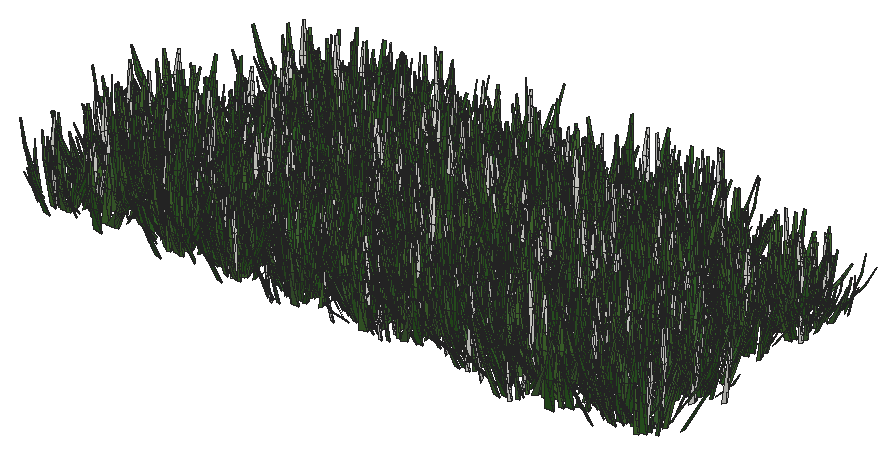
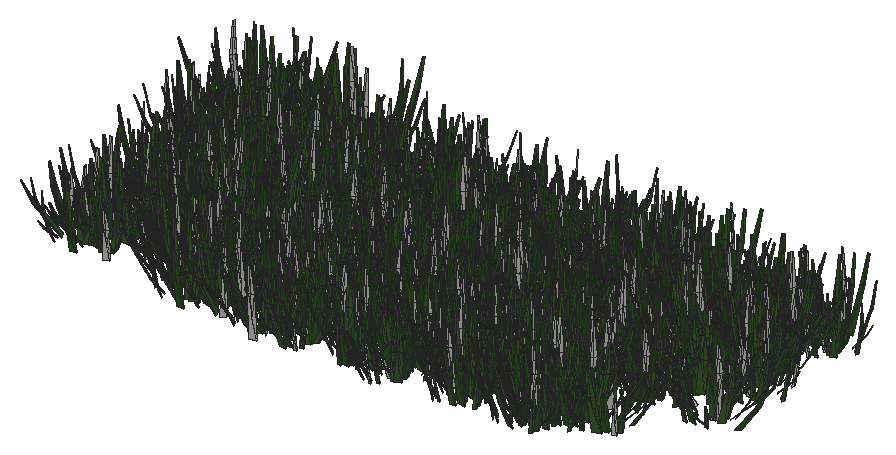
# SketchUp Ruby script. Lengths in inches.
U = 1.inch
M = Sketchup.active_model
def pt(a) = Geom::Point3d.new(a.map { |v| v * U })
def face(e, loops, mat)
  f = e.add_face(loops[0].map { |a| pt(a) })
  loops[1..].each { |l| e.add_face(l.map { |a| pt(a) }).erase! }
  f.material = f.back_material = mat if mat
  f
end
# faces: each face lists its corners as indices into pts; further lists are holes
def faces(e, pts, list, mat = nil) = list.each { |f| face(e, (f[0].is_a?(Array) ? f : [f]).map { |l| l.map { |i| pts[i] } }, mat) }
# xy, xz, yz: faces in a plane at the given z, y or x. An outline is a flat list of corners, or four numbers for a rectangle; further outlines are holes
def ring(l) = l.size == 4 ? [[l[0], l[1]], [l[2], l[1]], [l[2], l[3]], [l[0], l[3]]] : l.each_slice(2).to_a
def flat(e, list, mat, &to3) = list.each { |f| face(e, (f[0].is_a?(Array) ? f : [f]).map { |l| ring(l).map { |u, v| to3.(u, v) } }, mat) }
def xy(e, z, list, mat = nil) = flat(e, list, mat) { |x, y| [x, y, z] }
def xz(e, y, list, mat = nil) = flat(e, list, mat) { |x, z| [x, y, z] }
def yz(e, x, list, mat = nil) = flat(e, list, mat) { |y, z| [x, y, z] }
def lines(e, pts, list) = list.each { |a, b| e.add_line(pt(pts[a]), pt(pts[b])) }
# prism: a flat outline (further loops are holes) pulled along v
def prism(e, loops, v, mat = nil)
  f = face(e, loops, mat); d = Geom::Vector3d.new(v.map { |x| x * U })
  f.pushpull(f.normal.samedirection?(d) ? d.length : -d.length)
end
def box(e, o, s, mat = nil) = prism(e, [[o, [o[0] + s[0], o[1], o[2]], [o[0] + s[0], o[1] + s[1], o[2]], [o[0], o[1] + s[1], o[2]]]], [0, 0, s[2]], mat)
def at(x, y, z, deg = 0) = Geom::Transformation.translation(pt([x, y, z])) * Geom::Transformation.rotation(ORIGIN, Z_AXIS, deg.degrees)
def axes(o, x, y, z) = Geom::Transformation.new([*x, 0, *y, 0, *z, 0, *pt(o).to_a, 1])
def part(name) = M.definitions.add(name)
# library, detail: a bought-in or finely detailed component or shape, given as its bounding box
def library(name, o, s) = part(name).tap { |d| box(d.entities, o, s) }
def detail(e, o, s) = box(e.add_group.entities, o, s)
def put(e, d, t, mat = nil) = e.add_instance(d, t).tap { |i| i.material = mat if mat }
def group(e, t, mat = nil) = e.add_group.tap { |g| g.transformation = t; g.material = mat if mat }.entities
root = M.entities
M.materials.add("Material1").color = [58, 110, 58]
M.materials.add("Material10").color = [48, 100, 38]
M.materials.add("Material3").color = [68, 110, 58]
M.materials.add("Material4").color = [48, 90, 38]
M.materials.add("Material5").color = [68, 110, 48]
M.materials.add("Material6").color = [48, 90, 48]
M.materials.add("Material8").color = [58, 90, 38]
M.materials.add("Material9").color = [68, 100, 58]
c1 = part("grass00")
p = [[-0.6875,0.15,0],[-0.56,0.08,5.52],[-0.04,0.03,2.76],[0.48,-0.02,0],[0.35,-0.02,5.52],[-0.1,-0.14,5.52],
  [-0.12,0.65,8.37],[-0.42,0.65,8.37]]
faces(c1.entities,p,[[0,1,2,3],[3,2,4],[1,5,2],[5,4,2],[1,6,5],[4,5,6],[7,6,1]])
c2 = part("Group16\#1")
put(c2.entities,c1,axes([1.44,-0.61,-0.01],[0.05352,0.12609,0],[-0.10704,0.04543,0.07239],[0.06664,-0.02828,0.11628]),"Material6")
put(c2.entities,c1,axes([0.76,-0.15,-0.01],[0.04676,0.24062,0],[-0.23162,0.04501,0.06642],[0.0652,-0.01267,0.23595]),"Material3")
put(c2.entities,c1,axes([0.79,0.01,-0.01],[-0.00606,0.34651,0],[-0.34381,-0.00602,0.0432],[0.04319,0.00076,0.34386]))
put(c2.entities,c1,axes([1,0.23,-0.01],[-0.07192,0.31144,0],[-0.28722,-0.06632,0.1236],[0.12043,0.02781,0.29478]),"Material5")
put(c2.entities,c1,axes([1.66,0.77,-0.01],[-0.13828,0.29651,0],[-0.21551,-0.1005,0.22471],[0.20365,0.09498,0.23779]),"Material10")
put(c2.entities,c1,axes([0.6875,0.52,-0.01],[-0.18126,0.24051,0],[-0.22746,-0.17142,0.09788],[0.07817,0.05891,0.28481]),"Material5")
put(c2.entities,c1,axes([0.68,0.78,-0.01],[-0.215,0.18688,0],[-0.12385,-0.14248,0.21334],[0.13995,0.16101,0.18878]),"Material3")
put(c2.entities,c1,axes([0.56,1,-0.01],[-0.13756,0.07624,0],[-0.06159,-0.11112,0.0927],[0.04494,0.08108,0.12705]),"Material5")
put(c2.entities,c1,axes([0.2,0.64,-0.01],[-0.23729,0.07254,0],[-0.05711,-0.18681,0.153],[0.04473,0.14632,0.19535]),"Material10")
put(c2.entities,c1,axes([0.0625,0.72,-0.01],[-0.28874,0.02525,0],[-0.02179,-0.24916,0.14647],[0.01276,0.14591,0.25012]),"Material3")
put(c2.entities,c1,axes([-0.08,0.62,-0.01],[-0.34089,-0.04187,0],[0.03255,-0.26504,0.216],[-0.02633,0.21439,0.26703]),"Material10")
put(c2.entities,c1,axes([-0.34,0.98,-0.01],[-0.14314,-0.0493,0],[0.04397,-0.12769,0.06843],[-0.02228,0.0647,0.13505]),"Material10")
put(c2.entities,c1,axes([-0.87,1.45,-0.01],[-0.23488,-0.14114,0],[0.13761,-0.22901,0.06087],[-0.03135,0.05217,0.26717]))
put(c2.entities,c1,axes([-0.72,0.77,-0.01],[-0.14208,-0.13251,0],[0.07209,-0.0773,0.16301],[-0.11118,0.11922,0.1057]),"Material10")
put(c2.entities,c1,axes([-0.62,0.43,-0.01],[-0.14845,-0.21203,0],[0.18654,-0.13061,0.12304],[-0.10079,0.07057,0.22772]),"Material3")
put(c2.entities,c1,axes([-0.68,0.29,-0.01],[-0.13639,-0.32136,0],[0.31723,-0.13464,0.05579],[-0.05136,0.0218,0.34462]),"Material4")
put(c2.entities,c1,axes([-0.64,0.125,-0.01],[-0.0458,-0.23569,0],[0.22124,-0.043,0.08276],[-0.08124,0.01579,0.22538]),"Material1")
put(c2.entities,c1,axes([-1.6,-0.03,-0.01],[0.00576,-0.32897,0],[0.27526,0.00482,0.18018],[-0.18015,-0.00315,0.2753]),"Material5")
put(c2.entities,c1,axes([-1.36,-0.31,-0.01],[0.05718,-0.24765,0],[0.18172,0.04196,0.17267],[-0.16825,-0.03885,0.1865]),"Material10")
put(c2.entities,c1,axes([-1.54,-0.72,-0.01],[0.06537,-0.14017,0],[0.13555,0.06321,0.03939],[-0.0357,-0.01665,0.14956]))
put(c2.entities,c1,axes([-1.19,-0.9,-0.01],[0.09597,-0.12735,0],[0.11214,0.08451,0.07557],[-0.06035,-0.04548,0.14042]),"Material9")
put(c2.entities,c1,axes([-0.47,-0.54,-0.01],[0.11588,-0.10072,0],[0.0618,0.0711,0.12124],[-0.07953,-0.0915,0.0942]))
put(c2.entities,c1,axes([-0.47,-0.84,-0.01],[0.11927,-0.0661,0],[0.06603,0.11913,0.00646],[-0.00313,-0.00565,0.13621]),"Material5")
put(c2.entities,c1,axes([-0.38,-1.24,-0.01],[0.28037,-0.08571,0],[0.0618,0.20215,0.20315],[-0.05939,-0.19428,0.21139]),"Material9")
put(c2.entities,c1,axes([-0.06,-0.66,-0.01],[0.22719,-0.01987,0],[0.01247,0.14255,0.17758],[-0.01547,-0.17691,0.1431]),"Material8")
put(c2.entities,c1,axes([0.11,-0.89,-0.01],[0.14882,0.01828,0],[-0.01058,0.08611,0.12229],[0.01491,-0.12138,0.08676]),"Material6")
put(c2.entities,c1,axes([0.25,-0.72,-0.01],[0.20481,0.07053,0],[-0.06206,0.18022,0.10291],[0.03351,-0.0973,0.1906]),"Material6")
put(c2.entities,c1,axes([0.85,-1.42,-0.01],[0.16481,0.09904,0],[-0.09472,0.15762,0.05616],[0.02893,-0.04814,0.18389]),"Material5")
put(c2.entities,c1,axes([1.01,-1.09,-0.01],[0.21858,0.20385,0],[-0.17495,0.1876,0.15339],[0.10462,-0.11218,0.25652]),"Material10")
put(c2.entities,c1,axes([1.01,-0.71,-0.01],[0.08733,0.12473,0],[-0.06445,0.04512,0.13037],[0.1068,-0.07477,0.07867]),"Material6")
c3 = part("Group15\#1")
put(c3.entities,c2,at(0,0,0))
c4 = part("3darcstudiotree_grass00\#1")
put(c4.entities,c3,at(0,0,0))
put(root,c4,axes([325.61,114.35,0.25],[0.06749,1.02597,0],[-1.14616,0.05194,-0.05861],[-0.10032,0.00455,1.96776]))
put(root,c4,axes([312.01,114.49,0.25],[0.77982,0.60136,0],[-0.62193,0.5556,-0.03885],[-0.05655,0.05052,1.95422]))
put(root,c4,axes([308.2,114.68,0.25],[-0.48617,-0.67298,0],[0.85268,-0.42436,-0.04451],[0.05981,-0.02977,1.55797]))
put(root,c4,axes([297.52,114.8,0.25],[-0.43867,-0.79101,0],[0.90262,-0.34484,-0.04546],[0.07436,-0.02841,1.78943]))
put(root,c4,axes([299.75,114.88,0.25],[-0.15226,-0.79867,0],[1.26934,-0.16671,-0.05346],[0.06064,-0.00796,1.47567]))
put(root,c4,axes([327.16,115.04,0.25],[0.09684,-1.07066,0],[1.27143,0.07922,-0.06273],[0.09657,0.00602,1.9684]))
put(root,c4,axes([304.4,115,0.25],[-0.56509,-0.79358,0],[1.01126,-0.49607,-0.04139],[0.05602,-0.02748,1.84708]))
put(root,c4,axes([317.61,114.9,0.25],[0.41962,0.67368,0],[-1.06816,0.45834,-0.03477],[-0.04362,0.01872,1.69826]))
put(root,c4,axes([331.42,115.01,0.25],[-0.78759,-0.62837,0],[0.72827,-0.62883,-0.02949],[0.03824,-0.03302,1.96656]))
put(root,c4,axes([307.22,114.95,0.25],[-0.90146,-0.20082,0],[0.26222,-0.81085,-0.03217],[0.01535,-0.04746,1.86146]))
put(root,c4,axes([315.69,114.88,0.25],[-0.51566,0.71499,0],[-0.96817,-0.48104,-0.03562],[-0.03735,-0.01856,1.37892]))
put(root,c4,axes([322.51,115.05,0.25],[0.14547,0.81941,0],[-0.93806,0.11472,-0.04131],[-0.05805,0.0071,1.34689]))
put(root,c4,axes([328.45,115.42,0.25],[1.18815,-0.41208,0],[0.49804,0.98927,-0.05614],[0.02634,0.05231,1.57175]))
put(root,c4,axes([332.72,115.4,0.25],[0.99522,-0.21355,0],[0.28521,0.91566,-0.04398],[0.01824,0.05856,1.88821]))
put(root,c4,axes([303.94,115.41,0.25],[0.94192,-0.11841,0],[0.1867,1.02312,-0.05863],[0.01169,0.06407,1.66018]))
put(root,c4,axes([315.22,115.53,0.25],[0.91343,-0.26154,0],[0.30177,0.72606,-0.03311],[0.01837,0.04419,1.57439]))
put(root,c4,axes([311.33,115.66,0.25],[1.10887,0.19362,0],[-0.21686,0.85556,-0.04482],[-0.01325,0.05228,1.51278]))
put(root,c4,axes([318.83,115.875,0.25],[-0.20793,-0.75454,0],[1.14958,-0.21823,-0.04627],[0.07128,-0.01353,1.86363]))
put(root,c4,axes([316.27,115.99,0.25],[1.21024,0.36096,0],[-0.40297,0.93077,-0.03831],[-0.01666,0.03848,1.53223]))
put(root,c4,axes([320.33,115.9,0.25],[-0.98181,-0.4423,0],[0.58275,-0.89115,-0.04044],[0.02944,-0.04502,1.86421]))
put(root,c4,axes([313.12,116.17,0.25],[1.2003,0.24828,0],[-0.31214,1.03956,-0.03274],[-0.00995,0.03313,1.62193]))
put(root,c4,axes([308.18,116.07,0.25],[-0.67123,-0.59909,0],[0.68553,-0.52913,-0.03633],[0.04929,-0.03804,1.73438]))
put(root,c4,axes([324,116.23,0.25],[0.90739,0.27516,0],[-0.4147,0.9421,-0.04863],[-0.02152,0.0489,1.5585]))
put(root,c4,axes([301.62,116.3,0.25],[0.91927,0.31199,0],[-0.4318,0.87649,-0.03911],[-0.01951,0.03961,1.50402]))
put(root,c4,axes([329.5625,116.15,0.25],[-0.92811,-0.47122,0],[0.66196,-0.89818,-0.03935],[0.02332,-0.03164,1.44076]))
put(root,c4,axes([299.53,116.0625,0.25],[-0.92984,0.34747,0],[-0.49756,-0.91727,-0.05685],[-0.03628,-0.06688,1.88376]))
put(root,c4,axes([303.75,116.71,0.25],[0.92888,-0.1361,0],[0.20775,0.97682,-0.03701],[0.01068,0.05023,1.98432]))
put(root,c4,axes([319.51,116.93,0.25],[0.95404,0.51365,0],[-0.67211,0.86,-0.05832],[-0.03829,0.04899,1.48992]))
put(root,c4,axes([329.5,116.79,0.25],[0.18718,0.9905,0],[-0.92744,0.12074,-0.03929],[-0.08081,0.01052,1.95437]))
put(root,c4,axes([311.48,117.21,0.25],[0.87042,-0.41549,0],[0.61151,0.88252,-0.03788],[0.02157,0.03113,1.40078]))
put(root,c4,axes([325.13,117.1,0.25],[0.64918,0.69759,0],[-0.98053,0.62861,-0.04605],[-0.04237,0.02716,1.44046]))
put(root,c4,axes([306.77,116.99,0.25],[-0.04405,0.90565,0],[-1.17046,-0.03922,-0.04298],[-0.06922,-0.00232,1.88799]))
put(root,c4,axes([300.86,117.23,0.25],[0.25061,0.72688,0],[-1.19698,0.2843,-0.02742],[-0.041,0.00974,1.93645]))
put(root,c4,axes([305.36,117.21,0.25],[-1.06302,0.29862,0],[-0.29926,-0.73387,-0.02484],[-0.01679,-0.04118,1.96802]))
put(root,c4,axes([302.5,117.42,0.25],[0.61571,0.79749,0],[-1.07588,0.57223,-0.02786],[-0.03629,0.0193,1.9768]))
put(root,c4,axes([314.79,117.52,0.25],[-0.87953,-0.64988,0],[0.74058,-0.69046,-0.03256],[0.03159,-0.02945,1.62483]))
put(root,c4,axes([299.32,117.32,0.25],[-0.55611,0.84789,0],[-1.05997,-0.47894,-0.05406],[-0.06056,-0.02736,1.53936]))
put(root,c4,axes([318.07,117.5625,0.25],[-0.93845,-0.42279,0],[0.52303,-0.79979,-0.04387],[0.03253,-0.04974,1.70431]))
put(root,c4,axes([320.6,118.02,0.25],[-0.83191,-0.71207,0],[0.75763,-0.60977,-0.04714],[0.0509,-0.04097,1.58733]))
put(root,c4,axes([327.05,118.28,0.25],[0.55309,-0.68236,0],[1.0302,0.57526,-0.06298],[0.0561,0.03133,1.33293]))
put(root,c4,axes([331.46,118.16,0.25],[-0.81068,-0.80037,0],[0.75025,-0.5235,-0.02964],[0.03783,-0.0264,1.63454]))
put(root,c4,axes([302.28,118.17,0.25],[-0.9343,-0.567,0],[0.5485,-0.62264,-0.03203],[0.0397,-0.04507,1.95145]))
put(root,c4,axes([322.38,118.3,0.25],[0.88223,0.26687,0],[-0.44142,1.00529,-0.03532],[-0.01684,0.03836,1.79519]))
put(root,c4,axes([316.16,118,0.25],[-0.14808,0.93369,0],[-0.90663,-0.09906,-0.03263],[-0.05293,-0.00578,1.49628]))
put(root,c4,axes([317.57,118.08,0.25],[-1.22427,0.23578,0],[-0.22065,-0.78929,-0.03599],[-0.01197,-0.04283,1.43677]))
put(root,c4,axes([301.35,118.28,0.25],[-1.06365,-0.59761,0],[0.66853,-0.81972,-0.04034],[0.03082,-0.03779,1.62559]))
put(root,c4,axes([328.09,118.5,0.25],[1.07315,-0.42733,0],[0.44041,0.76193,-0.04597],[0.03081,0.0533,1.57738]))
put(root,c4,axes([306.98,118.49,0.25],[1.24229,0.07795,0],[-0.09135,1.00292,-0.04634],[-0.00573,0.06295,1.98901]))
put(root,c4,axes([308.29,118.5625,0.25],[1.1295,0.16862,0],[-0.19813,0.91428,-0.03729],[-0.00947,0.04371,1.60628]))
put(root,c4,axes([325.1875,118.6875,0.25],[1.04011,-0.60814,0],[0.60091,0.70802,-0.03692],[0.03742,0.04409,1.83631]))
put(root,c4,axes([310.44,118.58,0.25],[-0.91587,-0.75252,0],[0.89906,-0.75381,-0.03717],[0.0396,-0.0332,1.93537]))
put(root,c4,axes([329.77,118.67,0.25],[0.45288,0.69699,0],[-0.84077,0.37636,-0.03445],[-0.05836,0.02612,1.83855]))
put(root,c4,axes([304.63,118.78,0.25],[0.42612,0.68103,0],[-0.8909,0.38401,-0.04821],[-0.05831,0.02513,1.36797]))
put(root,c4,axes([298.08,119.18,0.25],[0.35164,0.85493,0],[-0.95508,0.27062,-0.04031],[-0.067,0.01898,1.77227]))
put(root,c4,axes([331.62,119.41,0.25],[1.06724,0.29906,0],[-0.40683,1.00015,-0.0473],[-0.02261,0.0556,1.90097]))
put(root,c4,axes([332.6,119.37,0.25],[-0.60586,-0.65224,0],[0.89762,-0.5744,-0.03514],[0.04334,-0.02773,1.76492]))
put(root,c4,axes([323.25,119.18,0.25],[-0.60419,0.6573,0],[-0.84601,-0.53573,-0.05103],[-0.06559,-0.04153,1.72023]))
put(root,c4,axes([316.13,119.59,0.25],[0.35122,-0.70599,0],[1.10902,0.38008,-0.04448],[0.06614,0.02267,1.93016]))
put(root,c4,axes([322.77,119.27,0.25],[0.15201,0.98728,0],[-0.95329,0.10112,-0.04145],[-0.08436,0.00895,1.97198]))
put(root,c4,axes([328.17,119.39,0.25],[-0.82248,0.44333,0],[-0.58974,-0.75373,-0.04277],[-0.0401,-0.05125,1.86401]))
put(root,c4,axes([311.63,119.8,0.25],[0.98051,-0.25756,0],[0.29084,0.76276,-0.04021],[0.01942,0.05094,1.5432]))
put(root,c4,axes([304.12,119.89,0.25],[1.27116,-0.01966,0],[0.0229,1.01998,-0.03615],[0.00085,0.03791,1.55355]))
put(root,c4,axes([301.08,120,0.25],[0.63022,-0.6463,0],[0.93622,0.62892,-0.0352],[0.04229,0.02841,1.86157]))
put(root,c4,axes([300.09,120.07,0.25],[1.03071,0.54196,0],[-0.59242,0.77616,-0.03414],[-0.0235,0.03079,1.42377]))
put(root,c4,axes([297.75,120.43,0.25],[-0.47078,-0.79062,0],[1.12869,-0.463,-0.04891],[0.06558,-0.0269,1.88309]))
put(root,c4,axes([319.26,120.76,0.25],[1.02181,-0.38725,0],[0.48911,0.8891,-0.05401],[0.02747,0.04993,1.44188]))
put(root,c4,axes([328.21,121.06,0.25],[0.89538,-0.15511,0],[0.19975,0.79435,-0.04941],[0.01501,0.05967,1.4533]))
put(root,c4,axes([314.43,120.96,0.25],[-0.96202,-0.52136,0],[0.58597,-0.74486,-0.0556],[0.04735,-0.06019,1.66946]))
put(root,c4,axes([323.84,120.79,0.25],[-0.07939,0.99944,0],[-0.91631,-0.05014,-0.03816],[-0.08086,-0.00442,1.95014]))
put(root,c4,axes([318.02,120.93,0.25],[0.743,0.83611,0],[-0.99495,0.6091,-0.05484],[-0.04692,0.02872,1.31443]))
put(root,c4,axes([300.63,121.32,0.25],[0.80537,-0.64063,0],[0.87207,0.75526,-0.03986],[0.03642,0.03154,1.66404]))
put(root,c4,axes([325.5625,121.34,0.25],[0.9128,-0.73982,0],[0.81134,0.68962,-0.04175],[0.0408,0.03468,1.62422]))
put(root,c4,axes([307.45,121.11,0.25],[0.73936,0.66919,0],[-0.66777,0.50826,-0.03804],[-0.05446,0.04145,1.7602]))
put(root,c4,axes([313.11,121.08,0.25],[-0.79004,0.55494,0],[-0.77146,-0.75661,-0.05904],[-0.04726,-0.04635,1.47981]))
put(root,c4,axes([310.17,121.08,0.25],[-0.86187,0.70731,0],[-0.70544,-0.59217,-0.03762],[-0.03878,-0.03255,1.47105]))
put(root,c4,axes([320.78,121.8,0.25],[0.60922,-0.56687,0],[0.89443,0.6622,-0.04874],[0.04371,0.03236,1.44038]))
put(root,c4,axes([303.73,121.74,0.25],[0.27921,0.72021,0],[-0.89646,0.23942,-0.0339],[-0.06201,0.01656,1.80984]))
put(root,c4,axes([324.35,121.7,0.25],[-0.6231,0.84686,0],[-1.05489,-0.5347,-0.0342],[-0.03865,-0.01959,1.63693]))
put(root,c4,axes([312.875,122.17,0.25],[-0.21887,-0.88537,0],[1.17151,-0.19951,-0.03341],[0.05094,-0.00867,1.86102]))
put(root,c4,axes([311.62,122.08,0.25],[-0.89815,-0.62334,0],[0.79766,-0.79177,-0.04137],[0.02922,-0.02901,1.36909]))
put(root,c4,axes([330.28,121.98,0.25],[-0.80456,0.51668,0],[-0.64053,-0.68711,-0.04163],[-0.03395,-0.03642,1.39503]))
put(root,c4,axes([307.43,122.2,0.25],[0.6287,0.61896,0],[-0.7039,0.49255,-0.04117],[-0.05307,0.03713,1.55213]))
put(root,c4,axes([310.12,122.31,0.25],[0.18402,0.74966,0],[-1.00864,0.17056,-0.04728],[-0.07397,0.01251,1.64346]))
put(root,c4,axes([328.14,122.2,0.25],[-0.96847,0.67158,0],[-0.70103,-0.69644,-0.03098],[-0.02897,-0.02878,1.59479]))
put(root,c4,axes([315.07,122.56,0.25],[-0.781,0.74115,0],[-0.9202,-0.66801,-0.03347],[-0.03945,-0.02864,1.91416]))
put(root,c4,axes([302.35,122.95,0.25],[1.25767,0.12703,0],[-0.14963,1.02059,-0.0359],[-0.00658,0.0449,1.88046]))
put(root,c4,axes([328.3,123.3,0.25],[1.10556,0.25176,0],[-0.29609,0.8957,-0.02738],[-0.01219,0.03689,1.88342]))
put(root,c4,axes([313.68,123.16,0.25],[0.47704,0.68147,0],[-0.89571,0.43195,-0.03711],[-0.05246,0.0253,1.69359]))
put(root,c4,axes([318.23,123.1,0.25],[0.04246,0.89262,0],[-1.29701,0.04251,-0.04149],[-0.04929,0.00162,1.54325]))
put(root,c4,axes([315.125,123.36,0.25],[-0.28465,-0.8073,0],[1.19901,-0.29124,-0.04795],[0.05642,-0.01371,1.53186]))
put(root,c4,axes([322.7,123.3,0.25],[1.00335,0.51632,0],[-0.54921,0.73523,-0.03504],[-0.0338,0.04525,1.90819]))
put(root,c4,axes([301.26,123.36,0.25],[-0.73601,-0.4972,0],[0.79538,-0.81113,-0.04334],[0.02916,-0.02974,1.34295]))
put(root,c4,axes([325.36,123.29,0.25],[-1.13116,0.1404,0],[-0.18956,-1.05213,-0.06496],[-0.01414,-0.07848,1.88637]))
put(root,c4,axes([309.09,123.68,0.25],[0.58262,-0.60834,0],[0.99031,0.65338,-0.06111],[0.06736,0.04444,1.78135]))
put(root,c4,axes([297.94,123.26,0.25],[-0.94247,0.69127,0],[-0.77842,-0.73112,-0.04086],[-0.03361,-0.03157,1.46035]))
put(root,c4,axes([319.04,123.7,0.25],[0.81865,-0.44426,0],[0.5025,0.63789,-0.045],[0.03682,0.04674,1.37282]))
put(root,c4,axes([316.76,123.45,0.25],[-0.58926,0.66001,0],[-0.93071,-0.57243,-0.05517],[-0.0662,-0.04072,1.72999]))
put(root,c4,axes([331.44,123.66,0.25],[0.68488,0.62152,0],[-0.81152,0.61605,-0.03451],[-0.0439,0.03332,1.89576]))
put(root,c4,axes([311.21,123.73,0.25],[-1.10567,-0.25203,0],[0.25953,-0.78436,-0.02848],[0.01413,-0.04269,1.83531]))
put(root,c4,axes([307.02,123.76,0.25],[0.37008,0.84448,0],[-1.19946,0.36212,-0.0524],[-0.0528,0.01594,1.36852]))
put(root,c4,axes([326.875,123.73,0.25],[-0.44773,0.66879,0],[-0.93335,-0.43045,-0.05151],[-0.08032,-0.03704,1.90487]))
put(root,c4,axes([316.2,124.43,0.25],[-0.08161,-0.89155,0],[1.14692,-0.07233,-0.05563],[0.09072,-0.00572,1.88098]))
put(root,c4,axes([304.48,124.24,0.25],[-1.17557,-0.07638,0],[0.09357,-0.99208,-0.05117],[0.00513,-0.0544,1.54048]))
put(root,c4,axes([319.49,124.49,0.25],[0.6721,0.57432,0],[-0.85997,0.69329,-0.03466],[-0.03938,0.03174,1.89896]))
put(root,c4,axes([328.1,124.7,0.25],[-0.09122,-0.80452,0],[0.95022,-0.07422,-0.04952],[0.06713,-0.00524,1.29958]))
put(root,c4,axes([306.03,124.64,0.25],[-1.22945,-0.16269,0],[0.16757,-0.87242,-0.05098],[0.01261,-0.06564,1.67187]))
put(root,c4,axes([331.32,124.71,0.25],[-0.63585,0.90167,0],[-1.00855,-0.48996,-0.03733],[-0.04095,-0.0199,1.48568]))
put(root,c4,axes([326.99,125.08,0.25],[-0.58565,-0.73336,0],[0.8931,-0.49133,-0.05028],[0.07623,-0.04194,1.94898]))
put(root,c4,axes([308.2,125.08,0.25],[0.89003,0.31258,0],[-0.38822,0.76153,-0.02719],[-0.02052,0.04025,1.929]))
put(root,c4,axes([312.15,125.74,0.25],[0.99499,-0.23487,0],[0.32617,0.95189,-0.03545],[0.01442,0.04208,1.77295]))
put(root,c4,axes([313.55,125.54,0.25],[-1.07459,-0.04214,0],[0.05884,-1.03383,-0.03065],[0.00228,-0.04013,1.9691]))
put(root,c4,axes([325.77,125.94,0.25],[-0.17255,-0.91357,0],[1.27507,-0.16591,-0.06318],[0.06747,-0.00878,1.39517]))
put(root,c4,axes([320.58,126.25,0.25],[0.96567,-0.06319,0],[0.10124,1.0658,-0.03935],[0.00347,0.03653,1.44542]))
put(root,c4,axes([309.94,125.9375,0.25],[-0.03163,0.83752,0],[-1.10227,-0.02868,-0.04067],[-0.05655,-0.00147,1.53414]))
put(root,c4,axes([327.32,126.13,0.25],[-0.80765,-0.82078,0],[0.97672,-0.6621,-0.03335],[0.03807,-0.02581,1.85855]))
put(root,c4,axes([304.67,126.02,0.25],[0.23134,0.73201,0],[-1.10289,0.24012,-0.05161],[-0.06656,0.01449,1.52021]))
put(root,c4,axes([319.65,126.03,0.25],[-0.01068,0.82642,0],[-1.02553,-0.00913,-0.03184],[-0.05324,-0.00047,1.71482]))
put(root,c4,axes([307.54,126.16,0.25],[-1.15861,-0.38506,0],[0.39187,-0.81229,-0.04264],[0.02541,-0.05267,1.69007]))
put(root,c4,axes([323.38,126.11,0.25],[-0.90994,0.64613,0],[-0.73942,-0.71737,-0.05065],[-0.04185,-0.0406,1.44592]))
put(root,c4,axes([318.97,126.71,0.25],[0.5764,-0.71336,0],[1.018,0.56665,-0.05795],[0.07632,0.04248,1.94389]))
put(root,c4,axes([320.51,126.8,0.25],[1.15803,-0.40217,0],[0.39877,0.79101,-0.04818],[0.02658,0.05272,1.47658]))
put(root,c4,axes([301.59,126.89,0.25],[0.4419,-0.92203,0],[1.19359,0.39408,-0.04298],[0.05253,0.01734,1.68954]))
put(root,c4,axes([318.31,126.79,0.25],[-1.16977,-0.17077,0],[0.21512,-1.01513,-0.04722],[0.00925,-0.04364,1.40384]))
put(root,c4,axes([327.9,127.17,0.25],[0.38578,-0.67655,0],[0.82368,0.32356,-0.04441],[0.08646,0.03396,1.96303]))
put(root,c4,axes([314.31,126.97,0.25],[-1.09096,0.03519,0],[-0.03666,-0.78286,-0.04521],[-0.00355,-0.07589,1.91035]))
put(root,c4,axes([311.13,127.22,0.25],[-0.10918,-1.03087,0],[1.09179,-0.07966,-0.04765],[0.07624,-0.00556,1.76037]))
put(root,c4,axes([330.83,127.1,0.25],[0.31184,0.95486,0],[-1.11523,0.25091,-0.03421],[-0.05538,0.01246,1.93796]))
put(root,c4,axes([332.44,127.12,0.25],[-0.37871,0.8877,0],[-0.87715,-0.2578,-0.04758],[-0.07594,-0.02232,1.57537]))
put(root,c4,axes([309.125,127.54,0.25],[0.95153,-0.36867,0],[0.49617,0.8822,-0.02938],[0.01747,0.03107,1.64954]))
put(root,c4,axes([307.27,127.55,0.25],[0.79074,-0.41612,0],[0.52624,0.6889,-0.03299],[0.03195,0.04182,1.77748]))
put(root,c4,axes([302.63,127.28,0.25],[-1.02548,0.62228,0],[-0.68997,-0.7833,-0.03994],[-0.03979,-0.04517,1.97331]))
put(root,c4,axes([304.16,127.47,0.25],[-0.69313,0.69872,0],[-0.79206,-0.54129,-0.04557],[-0.06355,-0.04343,1.85346]))
put(root,c4,axes([324.82,128.22,0.25],[0.00305,-0.83752,0],[1.24546,0.00312,-0.03692],[0.04678,0.00012,1.57831]))
put(root,c4,axes([305.23,128.29,0.25],[1.14599,0.16967,0],[-0.17112,0.79622,-0.04495],[-0.01603,0.07458,1.97854]))
put(root,c4,axes([326.67,128.35,0.25],[-0.52234,-0.82177,0],[0.95227,-0.41698,-0.03938],[0.04492,-0.01967,1.38871]))
put(root,c4,axes([331.08,128.43,0.25],[1.22401,0.06378,0],[-0.07206,0.95271,-0.04601],[-0.00329,0.04349,1.31249]))
put(root,c4,axes([319.71,128.31,0.25],[-0.9991,-0.43399,0],[0.53153,-0.84297,-0.05348],[0.03976,-0.06305,1.83786]))
put(root,c4,axes([316.29,128.24,0.25],[-0.26651,0.76981,0],[-1.2338,-0.29426,-0.06106],[-0.06734,-0.01606,1.47293]))
put(root,c4,axes([324.08,128.42,0.25],[-0.04195,0.85686,0],[-0.97768,-0.03297,-0.03031],[-0.0543,-0.00183,1.75443]))
put(root,c4,axes([303.67,128.6,0.25],[-0.68252,-0.5474,0],[0.7796,-0.66964,-0.03177],[0.03571,-0.03067,1.8145]))
put(root,c4,axes([332.4375,128.58,0.25],[-0.03629,0.96348,0],[-0.98658,-0.0256,-0.04056],[-0.05672,-0.00147,1.38085]))
put(root,c4,axes([308.34,128.76,0.25],[0.12651,0.81815,0],[-1.10446,0.11765,-0.0516],[-0.0918,0.00978,1.99718]))
put(root,c4,axes([318.19,128.89,0.25],[-1.20785,-0.05285,0],[0.06427,-1.01203,-0.0488],[0.00349,-0.05489,1.65721]))
put(root,c4,axes([319.76,129.22,0.25],[-1.156,0.2412,0],[-0.23565,-0.77802,-0.03206],[-0.01325,-0.04373,1.63785]))
put(root,c4,axes([304.58,129.41,0.25],[-0.87253,-0.27837,0],[0.39909,-0.86177,-0.04802],[0.02398,-0.05177,1.54794]))
put(root,c4,axes([318.08,129.75,0.25],[0.10313,-0.92577,0],[0.98093,0.07528,-0.04487],[0.06416,0.00492,1.41449]))
put(root,c4,axes([323.39,129.64,0.25],[1.04455,0.27707,0],[-0.31127,0.80843,-0.03842],[-0.02185,0.05674,1.90991]))
put(root,c4,axes([308.33,129.59,0.25],[-0.74973,-0.43064,0],[0.56451,-0.67704,-0.03348],[0.03599,-0.04317,1.87437]))
put(root,c4,axes([312.16,129.76,0.25],[-0.55357,-0.90648,0],[0.82911,-0.34881,-0.03791],[0.06862,-0.02887,1.88609]))
put(root,c4,axes([314.66,129.58,0.25],[-0.86427,0.47854,0],[-0.53226,-0.66223,-0.03251],[-0.03371,-0.04194,1.79208]))
put(root,c4,axes([320.42,130.01,0.25],[1.19713,-0.09326,0],[0.10677,0.94412,-0.03728],[0.0058,0.05131,1.90298]))
put(root,c4,axes([324.89,129.75,0.25],[0.03695,0.88657,0],[-1.02763,0.02951,-0.02489],[-0.04667,0.00134,1.9295]))
